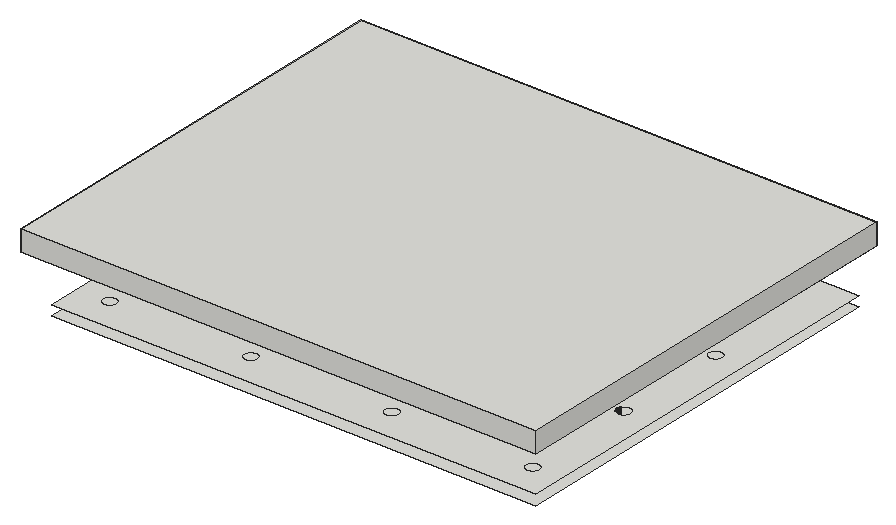
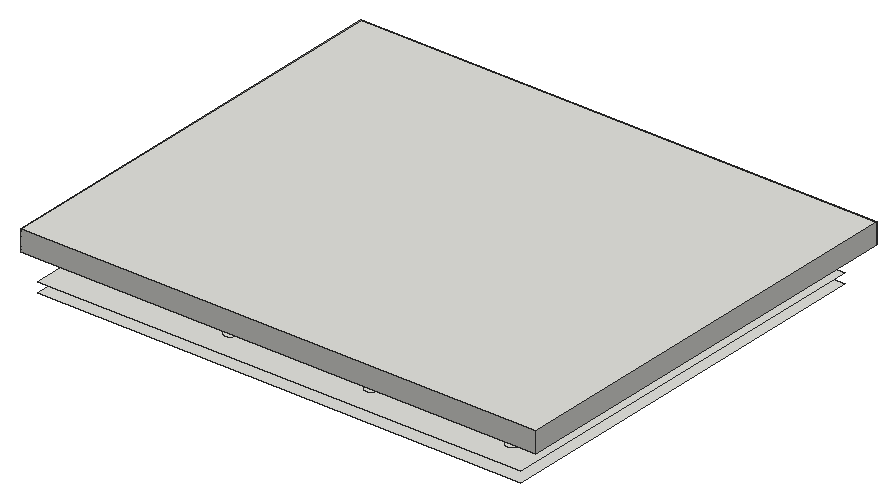
# SketchUp Ruby script. Lengths in millimetres.
U = 1.mm
M = Sketchup.active_model
def pt(a) = Geom::Point3d.new(a.map { |v| v * U })
def face(e, loops, mat)
  f = e.add_face(loops[0].map { |a| pt(a) })
  loops[1..].each { |l| e.add_face(l.map { |a| pt(a) }).erase! }
  f.material = f.back_material = mat if mat
  f
end
# faces: each face lists its corners as indices into pts; further lists are holes
def faces(e, pts, list, mat = nil) = list.each { |f| face(e, (f[0].is_a?(Array) ? f : [f]).map { |l| l.map { |i| pts[i] } }, mat) }
# xy, xz, yz: faces in a plane at the given z, y or x. An outline is a flat list of corners, or four numbers for a rectangle; further outlines are holes
def ring(l) = l.size == 4 ? [[l[0], l[1]], [l[2], l[1]], [l[2], l[3]], [l[0], l[3]]] : l.each_slice(2).to_a
def flat(e, list, mat, &to3) = list.each { |f| face(e, (f[0].is_a?(Array) ? f : [f]).map { |l| ring(l).map { |u, v| to3.(u, v) } }, mat) }
def xy(e, z, list, mat = nil) = flat(e, list, mat) { |x, y| [x, y, z] }
def xz(e, y, list, mat = nil) = flat(e, list, mat) { |x, z| [x, y, z] }
def yz(e, x, list, mat = nil) = flat(e, list, mat) { |y, z| [x, y, z] }
def lines(e, pts, list) = list.each { |a, b| e.add_line(pt(pts[a]), pt(pts[b])) }
# prism: a flat outline (further loops are holes) pulled along v
def prism(e, loops, v, mat = nil)
  f = face(e, loops, mat); d = Geom::Vector3d.new(v.map { |x| x * U })
  f.pushpull(f.normal.samedirection?(d) ? d.length : -d.length)
end
def box(e, o, s, mat = nil) = prism(e, [[o, [o[0] + s[0], o[1], o[2]], [o[0] + s[0], o[1] + s[1], o[2]], [o[0], o[1] + s[1], o[2]]]], [0, 0, s[2]], mat)
def at(x, y, z, deg = 0) = Geom::Transformation.translation(pt([x, y, z])) * Geom::Transformation.rotation(ORIGIN, Z_AXIS, deg.degrees)
def axes(o, x, y, z) = Geom::Transformation.new([*x, 0, *y, 0, *z, 0, *pt(o).to_a, 1])
def part(name) = M.definitions.add(name)
# library, detail: a bought-in or finely detailed component or shape, given as its bounding box
def library(name, o, s) = part(name).tap { |d| box(d.entities, o, s) }
def detail(e, o, s) = box(e.add_group.entities, o, s)
def put(e, d, t, mat = nil) = e.add_instance(d, t).tap { |i| i.material = mat if mat }
def group(e, t, mat = nil) = e.add_group.tap { |g| g.transformation = t; g.material = mat if mat }.entities
root = M.entities
c1 = part("Group\#21")
box(c1.entities,[-2669.7,0,0],[3683.6,3048,150])
xy(root,2718.2,[[[228.6,0,3683.6,2895.6],[685.8,457.2,3226.4,2438.4],[1465.5,177.8,1468.7,177.9,1471.9,178.2,1475.1,178.7,1478.2,179.4,1481.2,180.3,1484.2,181.4,1487.2,182.6,1490,184.1,1492.8,185.7,1495.4,187.5,1497.9,189.5,1500.3,191.6,1502.6,193.8,1504.7,196.2,1506.6,198.7,1508.4,201.4,1510,204.1,1511.5,207,1512.8,209.9,1513.8,212.9,1514.7,216,1515.4,219.1,1515.9,222.2,1516.2,225.4,1516.3,228.6,1516.2,231.8,1515.9,235,1515.4,238.1,1514.7,241.2,1513.8,244.3,1512.8,247.3,1511.5,250.2,1510,253.1,1508.4,255.8,1506.6,258.5,1504.7,261,1502.6,263.4,1500.3,265.6,1497.9,267.7,1495.4,269.7,1492.8,271.5,1490,273.1,1487.2,274.6,1484.2,275.8,1481.2,276.9,1478.2,277.8,1475.1,278.5,1471.9,279,1468.7,279.3,1465.5,279.4,1462.3,279.3,1459.2,279,1456,278.5,1452.9,277.8,1449.8,276.9,1446.8,275.8,1443.9,274.6,1441.1,273.1,1438.3,271.5,1435.7,269.7,1433.2,267.7,1430.8,265.6,1428.5,263.4,1426.4,261,1424.4,258.5,1422.6,255.8,1421,253.1,1419.6,250.2,1418.3,247.3,1417.2,244.3,1416.3,241.2,1415.6,238.1,1415.1,235,1414.8,231.8,1414.7,228.6,1414.8,225.4,1415.1,222.2,1415.6,219.1,1416.3,216,1417.2,212.9,1418.3,209.9,1419.6,207,1421,204.1,1422.6,201.4,1424.4,198.7,1426.4,196.2,1428.5,193.8,1430.8,191.6,1433.2,189.5,1435.7,187.5,1438.3,185.7,1441.1,184.1,1443.9,182.6,1446.8,181.4,1449.8,180.3,1452.9,179.4,1456,178.7,1459.2,178.2,1462.3,177.9],[457.2,177.8,460.4,177.9,463.6,178.2,466.7,178.7,469.8,179.4,472.9,180.3,475.9,181.4,478.8,182.6,481.7,184.1,484.4,185.7,487.1,187.5,489.6,189.5,492,191.6,494.2,193.8,496.3,196.2,498.3,198.7,500.1,201.4,501.7,204.1,503.2,207,504.4,209.9,505.5,212.9,506.4,216,507.1,219.1,507.6,222.2,507.9,225.4,508,228.6,507.9,231.8,507.6,235,507.1,238.1,506.4,241.2,505.5,244.3,504.4,247.3,503.2,250.2,501.7,253.1,500.1,255.8,498.3,258.5,496.3,261,494.2,263.4,492,265.6,489.6,267.7,487.1,269.7,484.4,271.5,481.7,273.1,478.8,274.6,475.9,275.8,472.9,276.9,469.8,277.8,466.7,278.5,463.6,279,460.4,279.3,457.2,279.4,454,279.3,450.8,279,447.7,278.5,444.6,277.8,441.5,276.9,438.5,275.8,435.6,274.6,432.7,273.1,430,271.5,427.3,269.7,424.8,267.7,422.4,265.6,420.2,263.4,418.1,261,416.1,258.5,414.3,255.8,412.7,253.1,411.2,250.2,410,247.3,408.9,244.3,408,241.2,407.3,238.1,406.8,235,406.5,231.8,406.4,228.6,406.5,225.4,406.8,222.2,407.3,219.1,408,216,408.9,212.9,410,209.9,411.2,207,412.7,204.1,414.3,201.4,416.1,198.7,418.1,196.2,420.2,193.8,422.4,191.6,424.8,189.5,427.3,187.5,430,185.7,432.7,184.1,435.6,182.6,438.5,181.4,441.5,180.3,444.6,179.4,447.7,178.7,450.8,178.2,454,177.9],[2473.9,177.8,2477.1,177.9,2480.2,178.2,2483.4,178.7,2486.5,179.4,2489.6,180.3,2492.6,181.4,2495.5,182.6,2498.3,184.1,2501.1,185.7,2503.7,187.5,2506.2,189.5,2508.6,191.6,2510.9,193.8,2513,196.2,2515,198.7,2516.8,201.4,2518.4,204.1,2519.8,207,2521.1,209.9,2522.2,212.9,2523.1,216,2523.8,219.1,2524.3,222.2,2524.6,225.4,2524.7,228.6,2524.6,231.8,2524.3,235,2523.8,238.1,2523.1,241.2,2522.2,244.3,2521.1,247.3,2519.8,250.2,2518.4,253.1,2516.8,255.8,2515,258.5,2513,261,2510.9,263.4,2508.6,265.6,2506.2,267.7,2503.7,269.7,2501.1,271.5,2498.3,273.1,2495.5,274.6,2492.6,275.8,2489.6,276.9,2486.5,277.8,2483.4,278.5,2480.2,279,2477.1,279.3,2473.9,279.4,2470.7,279.3,2467.5,279,2464.3,278.5,2461.2,277.8,2458.2,276.9,2455.2,275.8,2452.2,274.6,2449.4,273.1,2446.6,271.5,2444,269.7,2441.5,267.7,2439.1,265.6,2436.8,263.4,2434.7,261,2432.8,258.5,2431,255.8,2429.4,253.1,2427.9,250.2,2426.6,247.3,2425.6,244.3,2424.7,241.2,2424,238.1,2423.5,235,2423.2,231.8,2423.1,228.6,2423.2,225.4,2423.5,222.2,2424,219.1,2424.7,216,2425.6,212.9,2426.6,209.9,2427.9,207,2429.4,204.1,2431,201.4,2432.8,198.7,2434.7,196.2,2436.8,193.8,2439.1,191.6,2441.5,189.5,2444,187.5,2446.6,185.7,2449.4,184.1,2452.2,182.6,2455.2,181.4,2458.2,180.3,2461.2,179.4,2464.3,178.7,2467.5,178.2,2470.7,177.9],[3482.2,995.5,3485.4,995.6,3488.6,995.9,3491.7,996.4,3494.8,997.1,3497.9,998,3500.9,999,3503.8,1000.3,3506.7,1001.8,3509.4,1003.4,3512.1,1005.2,3514.6,1007.1,3517,1009.2,3519.2,1011.5,3521.3,1013.9,3523.3,1016.4,3525.1,1019,3526.7,1021.8,3528.2,1024.6,3529.4,1027.6,3530.5,1030.6,3531.4,1033.6,3532.1,1036.7,3532.6,1039.9,3532.9,1043.1,3533,1046.3,3532.9,1049.5,3532.6,1052.6,3532.1,1055.8,3531.4,1058.9,3530.5,1062,3529.4,1065,3528.2,1067.9,3526.7,1070.7,3525.1,1073.5,3523.3,1076.1,3521.3,1078.6,3519.2,1081,3517,1083.3,3514.6,1085.4,3512.1,1087.4,3509.4,1089.2,3506.7,1090.8,3503.8,1092.2,3500.9,1093.5,3497.9,1094.6,3494.8,1095.5,3491.7,1096.2,3488.6,1096.7,3485.4,1097,3482.2,1097.1,3479,1097,3475.8,1096.7,3472.7,1096.2,3469.6,1095.5,3466.5,1094.6,3463.5,1093.5,3460.6,1092.2,3457.7,1090.8,3455,1089.2,3452.3,1087.4,3449.8,1085.4,3447.4,1083.3,3445.2,1081,3443.1,1078.6,3441.1,1076.1,3439.3,1073.5,3437.7,1070.7,3436.2,1067.9,3435,1065,3433.9,1062,3433,1058.9,3432.3,1055.8,3431.8,1052.6,3431.5,1049.5,3431.4,1046.3,3431.5,1043.1,3431.8,1039.9,3432.3,1036.7,3433,1033.6,3433.9,1030.6,3435,1027.6,3436.2,1024.6,3437.7,1021.8,3439.3,1019,3441.1,1016.4,3443.1,1013.9,3445.2,1011.5,3447.4,1009.2,3449.8,1007.1,3452.3,1005.2,3455,1003.4,3457.7,1001.8,3460.6,1000.3,3463.5,999,3466.5,998,3469.6,997.1,3472.7,996.4,3475.8,995.9,3479,995.6],[457.2,1813.1,460.4,1813.2,463.6,1813.5,466.7,1814,469.8,1814.7,472.9,1815.6,475.9,1816.7,478.8,1818,481.7,1819.4,484.4,1821,487.1,1822.8,489.6,1824.8,492,1826.9,494.2,1829.2,496.3,1831.6,498.3,1834.1,500.1,1836.7,501.7,1839.5,503.2,1842.3,504.4,1845.2,505.5,1848.2,506.4,1851.3,507.1,1854.4,507.6,1857.6,507.9,1860.7,508,1863.9,507.9,1867.1,507.6,1870.3,507.1,1873.5,506.4,1876.6,505.5,1879.6,504.4,1882.6,503.2,1885.6,501.7,1888.4,500.1,1891.2,498.3,1893.8,496.3,1896.3,494.2,1898.7,492,1901,489.6,1903.1,487.1,1905,484.4,1906.8,481.7,1908.4,478.8,1909.9,475.9,1911.2,472.9,1912.2,469.8,1913.1,466.7,1913.8,463.6,1914.3,460.4,1914.6,457.2,1914.7,454,1914.6,450.8,1914.3,447.7,1913.8,444.6,1913.1,441.5,1912.2,438.5,1911.2,435.6,1909.9,432.7,1908.4,430,1906.8,427.3,1905,424.8,1903.1,422.4,1901,420.2,1898.7,418.1,1896.3,416.1,1893.8,414.3,1891.2,412.7,1888.4,411.2,1885.6,410,1882.6,408.9,1879.6,408,1876.6,407.3,1873.5,406.8,1870.3,406.5,1867.1,406.4,1863.9,406.5,1860.7,406.8,1857.6,407.3,1854.4,408,1851.3,408.9,1848.2,410,1845.2,411.2,1842.3,412.7,1839.5,414.3,1836.7,416.1,1834.1,418.1,1831.6,420.2,1829.2,422.4,1826.9,424.8,1824.8,427.3,1822.8,430,1821,432.7,1819.4,435.6,1818,438.5,1816.7,441.5,1815.6,444.6,1814.7,447.7,1814,450.8,1813.5,454,1813.2],[457.2,995.5,460.4,995.6,463.6,995.9,466.7,996.4,469.8,997.1,472.9,998,475.9,999,478.8,1000.3,481.7,1001.8,484.4,1003.4,487.1,1005.2,489.6,1007.1,492,1009.2,494.2,1011.5,496.3,1013.9,498.3,1016.4,500.1,1019,501.7,1021.8,503.2,1024.6,504.4,1027.6,505.5,1030.6,506.4,1033.6,507.1,1036.7,507.6,1039.9,507.9,1043.1,508,1046.3,507.9,1049.5,507.6,1052.6,507.1,1055.8,506.4,1058.9,505.5,1062,504.4,1065,503.2,1067.9,501.7,1070.7,500.1,1073.5,498.3,1076.1,496.3,1078.6,494.2,1081,492,1083.3,489.6,1085.4,487.1,1087.4,484.4,1089.2,481.7,1090.8,478.8,1092.2,475.9,1093.5,472.9,1094.6,469.8,1095.5,466.7,1096.2,463.6,1096.7,460.4,1097,457.2,1097.1,454,1097,450.8,1096.7,447.7,1096.2,444.6,1095.5,441.5,1094.6,438.5,1093.5,435.6,1092.2,432.7,1090.8,430,1089.2,427.3,1087.4,424.8,1085.4,422.4,1083.3,420.2,1081,418.1,1078.6,416.1,1076.1,414.3,1073.5,412.7,1070.7,411.2,1067.9,410,1065,408.9,1062,408,1058.9,407.3,1055.8,406.8,1052.6,406.5,1049.5,406.4,1046.3,406.5,1043.1,406.8,1039.9,407.3,1036.7,408,1033.6,408.9,1030.6,410,1027.6,411.2,1024.6,412.7,1021.8,414.3,1019,416.1,1016.4,418.1,1013.9,420.2,1011.5,422.4,1009.2,424.8,1007.1,427.3,1005.2,430,1003.4,432.7,1001.8,435.6,1000.3,438.5,999,441.5,998,444.6,997.1,447.7,996.4,450.8,995.9,454,995.6],[3482.2,177.8,3485.4,177.9,3488.6,178.2,3491.7,178.7,3494.8,179.4,3497.9,180.3,3500.9,181.4,3503.8,182.6,3506.7,184.1,3509.4,185.7,3512.1,187.5,3514.6,189.5,3517,191.6,3519.2,193.8,3521.3,196.2,3523.3,198.7,3525.1,201.4,3526.7,204.1,3528.2,207,3529.4,209.9,3530.5,212.9,3531.4,216,3532.1,219.1,3532.6,222.2,3532.9,225.4,3533,228.6,3532.9,231.8,3532.6,235,3532.1,238.1,3531.4,241.2,3530.5,244.3,3529.4,247.3,3528.2,250.2,3526.7,253.1,3525.1,255.8,3523.3,258.5,3521.3,261,3519.2,263.4,3517,265.6,3514.6,267.7,3512.1,269.7,3509.4,271.5,3506.7,273.1,3503.8,274.6,3500.9,275.8,3497.9,276.9,3494.8,277.8,3491.7,278.5,3488.6,279,3485.4,279.3,3482.2,279.4,3479,279.3,3475.8,279,3472.7,278.5,3469.6,277.8,3466.5,276.9,3463.5,275.8,3460.6,274.6,3457.7,273.1,3455,271.5,3452.3,269.7,3449.8,267.7,3447.4,265.6,3445.2,263.4,3443.1,261,3441.1,258.5,3439.3,255.8,3437.7,253.1,3436.2,250.2,3435,247.3,3433.9,244.3,3433,241.2,3432.3,238.1,3431.8,235,3431.5,231.8,3431.4,228.6,3431.5,225.4,3431.8,222.2,3432.3,219.1,3433,216,3433.9,212.9,3435,209.9,3436.2,207,3437.7,204.1,3439.3,201.4,3441.1,198.7,3443.1,196.2,3445.2,193.8,3447.4,191.6,3449.8,189.5,3452.3,187.5,3455,185.7,3457.7,184.1,3460.6,182.6,3463.5,181.4,3466.5,180.3,3469.6,179.4,3472.7,178.7,3475.8,178.2,3479,177.9],[457.2,2630.8,460.4,2630.9,463.6,2631.2,466.7,2631.7,469.8,2632.4,472.9,2633.3,475.9,2634.4,478.8,2635.6,481.7,2637.1,484.4,2638.7,487.1,2640.5,489.6,2642.5,492,2644.6,494.2,2646.8,496.3,2649.2,498.3,2651.7,500.1,2654.4,501.7,2657.1,503.2,2660,504.4,2662.9,505.5,2665.9,506.4,2669,507.1,2672.1,507.6,2675.2,507.9,2678.4,508,2681.6,507.9,2684.8,507.6,2688,507.1,2691.1,506.4,2694.2,505.5,2697.3,504.4,2700.3,503.2,2703.2,501.7,2706.1,500.1,2708.8,498.3,2711.5,496.3,2714,494.2,2716.4,492,2718.6,489.6,2720.7,487.1,2722.7,484.4,2724.5,481.7,2726.1,478.8,2727.6,475.9,2728.8,472.9,2729.9,469.8,2730.8,466.7,2731.5,463.6,2732,460.4,2732.3,457.2,2732.4,454,2732.3,450.8,2732,447.7,2731.5,444.6,2730.8,441.5,2729.9,438.5,2728.8,435.6,2727.6,432.7,2726.1,430,2724.5,427.3,2722.7,424.8,2720.7,422.4,2718.6,420.2,2716.4,418.1,2714,416.1,2711.5,414.3,2708.8,412.7,2706.1,411.2,2703.2,410,2700.3,408.9,2697.3,408,2694.2,407.3,2691.1,406.8,2688,406.5,2684.8,406.4,2681.6,406.5,2678.4,406.8,2675.2,407.3,2672.1,408,2669,408.9,2665.9,410,2662.9,411.2,2660,412.7,2657.1,414.3,2654.4,416.1,2651.7,418.1,2649.2,420.2,2646.8,422.4,2644.6,424.8,2642.5,427.3,2640.5,430,2638.7,432.7,2637.1,435.6,2635.6,438.5,2634.4,441.5,2633.3,444.6,2632.4,447.7,2631.7,450.8,2631.2,454,2630.9],[2473.9,2630.8,2477.1,2630.9,2480.2,2631.2,2483.4,2631.7,2486.5,2632.4,2489.6,2633.3,2492.6,2634.4,2495.5,2635.6,2498.3,2637.1,2501.1,2638.7,2503.7,2640.5,2506.2,2642.5,2508.6,2644.6,2510.9,2646.8,2513,2649.2,2515,2651.7,2516.8,2654.4,2518.4,2657.1,2519.8,2660,2521.1,2662.9,2522.2,2665.9,2523.1,2669,2523.8,2672.1,2524.3,2675.2,2524.6,2678.4,2524.7,2681.6,2524.6,2684.8,2524.3,2688,2523.8,2691.1,2523.1,2694.2,2522.2,2697.3,2521.1,2700.3,2519.8,2703.2,2518.4,2706.1,2516.8,2708.8,2515,2711.5,2513,2714,2510.9,2716.4,2508.6,2718.6,2506.2,2720.7,2503.7,2722.7,2501.1,2724.5,2498.3,2726.1,2495.5,2727.6,2492.6,2728.8,2489.6,2729.9,2486.5,2730.8,2483.4,2731.5,2480.2,2732,2477.1,2732.3,2473.9,2732.4,2470.7,2732.3,2467.5,2732,2464.3,2731.5,2461.2,2730.8,2458.2,2729.9,2455.2,2728.8,2452.2,2727.6,2449.4,2726.1,2446.6,2724.5,2444,2722.7,2441.5,2720.7,2439.1,2718.6,2436.8,2716.4,2434.7,2714,2432.8,2711.5,2431,2708.8,2429.4,2706.1,2427.9,2703.2,2426.6,2700.3,2425.6,2697.3,2424.7,2694.2,2424,2691.1,2423.5,2688,2423.2,2684.8,2423.1,2681.6,2423.2,2678.4,2423.5,2675.2,2424,2672.1,2424.7,2669,2425.6,2665.9,2426.6,2662.9,2427.9,2660,2429.4,2657.1,2431,2654.4,2432.8,2651.7,2434.7,2649.2,2436.8,2646.8,2439.1,2644.6,2441.5,2642.5,2444,2640.5,2446.6,2638.7,2449.4,2637.1,2452.2,2635.6,2455.2,2634.4,2458.2,2633.3,2461.2,2632.4,2464.3,2631.7,2467.5,2631.2,2470.7,2630.9],[1465.5,2630.8,1468.7,2630.9,1471.9,2631.2,1475.1,2631.7,1478.2,2632.4,1481.2,2633.3,1484.2,2634.4,1487.2,2635.6,1490,2637.1,1492.8,2638.7,1495.4,2640.5,1497.9,2642.5,1500.3,2644.6,1502.6,2646.8,1504.7,2649.2,1506.6,2651.7,1508.4,2654.4,1510,2657.1,1511.5,2660,1512.8,2662.9,1513.8,2665.9,1514.7,2669,1515.4,2672.1,1515.9,2675.2,1516.2,2678.4,1516.3,2681.6,1516.2,2684.8,1515.9,2688,1515.4,2691.1,1514.7,2694.2,1513.8,2697.3,1512.8,2700.3,1511.5,2703.2,1510,2706.1,1508.4,2708.8,1506.6,2711.5,1504.7,2714,1502.6,2716.4,1500.3,2718.6,1497.9,2720.7,1495.4,2722.7,1492.8,2724.5,1490,2726.1,1487.2,2727.6,1484.2,2728.8,1481.2,2729.9,1478.2,2730.8,1475.1,2731.5,1471.9,2732,1468.7,2732.3,1465.5,2732.4,1462.3,2732.3,1459.2,2732,1456,2731.5,1452.9,2730.8,1449.8,2729.9,1446.8,2728.8,1443.9,2727.6,1441.1,2726.1,1438.3,2724.5,1435.7,2722.7,1433.2,2720.7,1430.8,2718.6,1428.5,2716.4,1426.4,2714,1424.4,2711.5,1422.6,2708.8,1421,2706.1,1419.6,2703.2,1418.3,2700.3,1417.2,2697.3,1416.3,2694.2,1415.6,2691.1,1415.1,2688,1414.8,2684.8,1414.7,2681.6,1414.8,2678.4,1415.1,2675.2,1415.6,2672.1,1416.3,2669,1417.2,2665.9,1418.3,2662.9,1419.6,2660,1421,2657.1,1422.6,2654.4,1424.4,2651.7,1426.4,2649.2,1428.5,2646.8,1430.8,2644.6,1433.2,2642.5,1435.7,2640.5,1438.3,2638.7,1441.1,2637.1,1443.9,2635.6,1446.8,2634.4,1449.8,2633.3,1452.9,2632.4,1456,2631.7,1459.2,2631.2,1462.3,2630.9],[3482.2,1813.1,3485.4,1813.2,3488.6,1813.5,3491.7,1814,3494.8,1814.7,3497.9,1815.6,3500.9,1816.7,3503.8,1818,3506.7,1819.4,3509.4,1821,3512.1,1822.8,3514.6,1824.8,3517,1826.9,3519.2,1829.2,3521.3,1831.6,3523.3,1834.1,3525.1,1836.7,3526.7,1839.5,3528.2,1842.3,3529.4,1845.2,3530.5,1848.2,3531.4,1851.3,3532.1,1854.4,3532.6,1857.6,3532.9,1860.7,3533,1863.9,3532.9,1867.1,3532.6,1870.3,3532.1,1873.5,3531.4,1876.6,3530.5,1879.6,3529.4,1882.6,3528.2,1885.6,3526.7,1888.4,3525.1,1891.2,3523.3,1893.8,3521.3,1896.3,3519.2,1898.7,3517,1901,3514.6,1903.1,3512.1,1905,3509.4,1906.8,3506.7,1908.4,3503.8,1909.9,3500.9,1911.2,3497.9,1912.2,3494.8,1913.1,3491.7,1913.8,3488.6,1914.3,3485.4,1914.6,3482.2,1914.7,3479,1914.6,3475.8,1914.3,3472.7,1913.8,3469.6,1913.1,3466.5,1912.2,3463.5,1911.2,3460.6,1909.9,3457.7,1908.4,3455,1906.8,3452.3,1905,3449.8,1903.1,3447.4,1901,3445.2,1898.7,3443.1,1896.3,3441.1,1893.8,3439.3,1891.2,3437.7,1888.4,3436.2,1885.6,3435,1882.6,3433.9,1879.6,3433,1876.6,3432.3,1873.5,3431.8,1870.3,3431.5,1867.1,3431.4,1863.9,3431.5,1860.7,3431.8,1857.6,3432.3,1854.4,3433,1851.3,3433.9,1848.2,3435,1845.2,3436.2,1842.3,3437.7,1839.5,3439.3,1836.7,3441.1,1834.1,3443.1,1831.6,3445.2,1829.2,3447.4,1826.9,3449.8,1824.8,3452.3,1822.8,3455,1821,3457.7,1819.4,3460.6,1818,3463.5,1816.7,3466.5,1815.6,3469.6,1814.7,3472.7,1814,3475.8,1813.5,3479,1813.2]]])
xy(root,2743.2,[[[635,406.4,3277.2,2489.2],[673.1,444.5,3239.1,2451.1]],[[1003.3,774.7,2908.9,2120.9],[1041.4,812.8,2870.8,2082.8]]])
xy(root,2766.6,[[[673.1,444.5,3239.1,2451.1],[685.8,457.2,3226.4,2438.4]]])
xy(root,2768.6,[[[990.6,762,2921.6,2133.6],[1003.3,774.7,2908.9,2120.9]]])
xy(root,2794,[[[228.6,0,3683.6,2895.6],[635,406.4,3277.2,2489.2],[457.2,1813.1,454,1813.2,450.8,1813.5,447.7,1814,444.6,1814.7,441.5,1815.6,438.5,1816.7,435.6,1818,432.7,1819.4,430,1821,427.3,1822.8,424.8,1824.8,422.4,1826.9,420.2,1829.2,418.1,1831.6,416.1,1834.1,414.3,1836.7,412.7,1839.5,411.2,1842.3,410,1845.2,408.9,1848.2,408,1851.3,407.3,1854.4,406.8,1857.6,406.5,1860.7,406.4,1863.9,406.5,1867.1,406.8,1870.3,407.3,1873.5,408,1876.6,408.9,1879.6,410,1882.6,411.2,1885.6,412.7,1888.4,414.3,1891.2,416.1,1893.8,418.1,1896.3,420.2,1898.7,422.4,1901,424.8,1903.1,427.3,1905,430,1906.8,432.7,1908.4,435.6,1909.9,438.5,1911.2,441.5,1912.2,444.6,1913.1,447.7,1913.8,450.8,1914.3,454,1914.6,457.2,1914.7,460.4,1914.6,463.6,1914.3,466.7,1913.8,469.8,1913.1,472.9,1912.2,475.9,1911.2,478.8,1909.9,481.7,1908.4,484.4,1906.8,487.1,1905,489.6,1903.1,492,1901,494.2,1898.7,496.3,1896.3,498.3,1893.8,500.1,1891.2,501.7,1888.4,503.2,1885.6,504.4,1882.6,505.5,1879.6,506.4,1876.6,507.1,1873.5,507.6,1870.3,507.9,1867.1,508,1863.9,507.9,1860.7,507.6,1857.6,507.1,1854.4,506.4,1851.3,505.5,1848.2,504.4,1845.2,503.2,1842.3,501.7,1839.5,500.1,1836.7,498.3,1834.1,496.3,1831.6,494.2,1829.2,492,1826.9,489.6,1824.8,487.1,1822.8,484.4,1821,481.7,1819.4,478.8,1818,475.9,1816.7,472.9,1815.6,469.8,1814.7,466.7,1814,463.6,1813.5,460.4,1813.2],[3482.2,177.8,3479,177.9,3475.8,178.2,3472.7,178.7,3469.6,179.4,3466.5,180.3,3463.5,181.4,3460.6,182.6,3457.7,184.1,3455,185.7,3452.3,187.5,3449.8,189.5,3447.4,191.6,3445.2,193.8,3443.1,196.2,3441.1,198.7,3439.3,201.4,3437.7,204.1,3436.2,207,3435,209.9,3433.9,212.9,3433,216,3432.3,219.1,3431.8,222.2,3431.5,225.4,3431.4,228.6,3431.5,231.8,3431.8,235,3432.3,238.1,3433,241.2,3433.9,244.3,3435,247.3,3436.2,250.2,3437.7,253.1,3439.3,255.8,3441.1,258.5,3443.1,261,3445.2,263.4,3447.4,265.6,3449.8,267.7,3452.3,269.7,3455,271.5,3457.7,273.1,3460.6,274.6,3463.5,275.8,3466.5,276.9,3469.6,277.8,3472.7,278.5,3475.8,279,3479,279.3,3482.2,279.4,3485.4,279.3,3488.6,279,3491.7,278.5,3494.8,277.8,3497.9,276.9,3500.9,275.8,3503.8,274.6,3506.7,273.1,3509.4,271.5,3512.1,269.7,3514.6,267.7,3517,265.6,3519.2,263.4,3521.3,261,3523.3,258.5,3525.1,255.8,3526.7,253.1,3528.2,250.2,3529.4,247.3,3530.5,244.3,3531.4,241.2,3532.1,238.1,3532.6,235,3532.9,231.8,3533,228.6,3532.9,225.4,3532.6,222.2,3532.1,219.1,3531.4,216,3530.5,212.9,3529.4,209.9,3528.2,207,3526.7,204.1,3525.1,201.4,3523.3,198.7,3521.3,196.2,3519.2,193.8,3517,191.6,3514.6,189.5,3512.1,187.5,3509.4,185.7,3506.7,184.1,3503.8,182.6,3500.9,181.4,3497.9,180.3,3494.8,179.4,3491.7,178.7,3488.6,178.2,3485.4,177.9],[457.2,177.8,454,177.9,450.8,178.2,447.7,178.7,444.6,179.4,441.5,180.3,438.5,181.4,435.6,182.6,432.7,184.1,430,185.7,427.3,187.5,424.8,189.5,422.4,191.6,420.2,193.8,418.1,196.2,416.1,198.7,414.3,201.4,412.7,204.1,411.2,207,410,209.9,408.9,212.9,408,216,407.3,219.1,406.8,222.2,406.5,225.4,406.4,228.6,406.5,231.8,406.8,235,407.3,238.1,408,241.2,408.9,244.3,410,247.3,411.2,250.2,412.7,253.1,414.3,255.8,416.1,258.5,418.1,261,420.2,263.4,422.4,265.6,424.8,267.7,427.3,269.7,430,271.5,432.7,273.1,435.6,274.6,438.5,275.8,441.5,276.9,444.6,277.8,447.7,278.5,450.8,279,454,279.3,457.2,279.4,460.4,279.3,463.6,279,466.7,278.5,469.8,277.8,472.9,276.9,475.9,275.8,478.8,274.6,481.7,273.1,484.4,271.5,487.1,269.7,489.6,267.7,492,265.6,494.2,263.4,496.3,261,498.3,258.5,500.1,255.8,501.7,253.1,503.2,250.2,504.4,247.3,505.5,244.3,506.4,241.2,507.1,238.1,507.6,235,507.9,231.8,508,228.6,507.9,225.4,507.6,222.2,507.1,219.1,506.4,216,505.5,212.9,504.4,209.9,503.2,207,501.7,204.1,500.1,201.4,498.3,198.7,496.3,196.2,494.2,193.8,492,191.6,489.6,189.5,487.1,187.5,484.4,185.7,481.7,184.1,478.8,182.6,475.9,181.4,472.9,180.3,469.8,179.4,466.7,178.7,463.6,178.2,460.4,177.9],[1465.5,177.8,1462.3,177.9,1459.2,178.2,1456,178.7,1452.9,179.4,1449.8,180.3,1446.8,181.4,1443.9,182.6,1441.1,184.1,1438.3,185.7,1435.7,187.5,1433.2,189.5,1430.8,191.6,1428.5,193.8,1426.4,196.2,1424.4,198.7,1422.6,201.4,1421,204.1,1419.6,207,1418.3,209.9,1417.2,212.9,1416.3,216,1415.6,219.1,1415.1,222.2,1414.8,225.4,1414.7,228.6,1414.8,231.8,1415.1,235,1415.6,238.1,1416.3,241.2,1417.2,244.3,1418.3,247.3,1419.6,250.2,1421,253.1,1422.6,255.8,1424.4,258.5,1426.4,261,1428.5,263.4,1430.8,265.6,1433.2,267.7,1435.7,269.7,1438.3,271.5,1441.1,273.1,1443.9,274.6,1446.8,275.8,1449.8,276.9,1452.9,277.8,1456,278.5,1459.2,279,1462.3,279.3,1465.5,279.4,1468.7,279.3,1471.9,279,1475.1,278.5,1478.2,277.8,1481.2,276.9,1484.2,275.8,1487.2,274.6,1490,273.1,1492.8,271.5,1495.4,269.7,1497.9,267.7,1500.3,265.6,1502.6,263.4,1504.7,261,1506.6,258.5,1508.4,255.8,1510,253.1,1511.5,250.2,1512.8,247.3,1513.8,244.3,1514.7,241.2,1515.4,238.1,1515.9,235,1516.2,231.8,1516.3,228.6,1516.2,225.4,1515.9,222.2,1515.4,219.1,1514.7,216,1513.8,212.9,1512.8,209.9,1511.5,207,1510,204.1,1508.4,201.4,1506.6,198.7,1504.7,196.2,1502.6,193.8,1500.3,191.6,1497.9,189.5,1495.4,187.5,1492.8,185.7,1490,184.1,1487.2,182.6,1484.2,181.4,1481.2,180.3,1478.2,179.4,1475.1,178.7,1471.9,178.2,1468.7,177.9],[2473.9,177.8,2470.7,177.9,2467.5,178.2,2464.3,178.7,2461.2,179.4,2458.2,180.3,2455.2,181.4,2452.2,182.6,2449.4,184.1,2446.6,185.7,2444,187.5,2441.5,189.5,2439.1,191.6,2436.8,193.8,2434.7,196.2,2432.8,198.7,2431,201.4,2429.4,204.1,2427.9,207,2426.6,209.9,2425.6,212.9,2424.7,216,2424,219.1,2423.5,222.2,2423.2,225.4,2423.1,228.6,2423.2,231.8,2423.5,235,2424,238.1,2424.7,241.2,2425.6,244.3,2426.6,247.3,2427.9,250.2,2429.4,253.1,2431,255.8,2432.8,258.5,2434.7,261,2436.8,263.4,2439.1,265.6,2441.5,267.7,2444,269.7,2446.6,271.5,2449.4,273.1,2452.2,274.6,2455.2,275.8,2458.2,276.9,2461.2,277.8,2464.3,278.5,2467.5,279,2470.7,279.3,2473.9,279.4,2477.1,279.3,2480.2,279,2483.4,278.5,2486.5,277.8,2489.6,276.9,2492.6,275.8,2495.5,274.6,2498.3,273.1,2501.1,271.5,2503.7,269.7,2506.2,267.7,2508.6,265.6,2510.9,263.4,2513,261,2515,258.5,2516.8,255.8,2518.4,253.1,2519.8,250.2,2521.1,247.3,2522.2,244.3,2523.1,241.2,2523.8,238.1,2524.3,235,2524.6,231.8,2524.7,228.6,2524.6,225.4,2524.3,222.2,2523.8,219.1,2523.1,216,2522.2,212.9,2521.1,209.9,2519.8,207,2518.4,204.1,2516.8,201.4,2515,198.7,2513,196.2,2510.9,193.8,2508.6,191.6,2506.2,189.5,2503.7,187.5,2501.1,185.7,2498.3,184.1,2495.5,182.6,2492.6,181.4,2489.6,180.3,2486.5,179.4,2483.4,178.7,2480.2,178.2,2477.1,177.9],[2473.9,2630.8,2470.7,2630.9,2467.5,2631.2,2464.3,2631.7,2461.2,2632.4,2458.2,2633.3,2455.2,2634.4,2452.2,2635.6,2449.4,2637.1,2446.6,2638.7,2444,2640.5,2441.5,2642.5,2439.1,2644.6,2436.8,2646.8,2434.7,2649.2,2432.8,2651.7,2431,2654.4,2429.4,2657.1,2427.9,2660,2426.6,2662.9,2425.6,2665.9,2424.7,2669,2424,2672.1,2423.5,2675.2,2423.2,2678.4,2423.1,2681.6,2423.2,2684.8,2423.5,2688,2424,2691.1,2424.7,2694.2,2425.6,2697.3,2426.6,2700.3,2427.9,2703.2,2429.4,2706.1,2431,2708.8,2432.8,2711.5,2434.7,2714,2436.8,2716.4,2439.1,2718.6,2441.5,2720.7,2444,2722.7,2446.6,2724.5,2449.4,2726.1,2452.2,2727.6,2455.2,2728.8,2458.2,2729.9,2461.2,2730.8,2464.3,2731.5,2467.5,2732,2470.7,2732.3,2473.9,2732.4,2477.1,2732.3,2480.2,2732,2483.4,2731.5,2486.5,2730.8,2489.6,2729.9,2492.6,2728.8,2495.5,2727.6,2498.3,2726.1,2501.1,2724.5,2503.7,2722.7,2506.2,2720.7,2508.6,2718.6,2510.9,2716.4,2513,2714,2515,2711.5,2516.8,2708.8,2518.4,2706.1,2519.8,2703.2,2521.1,2700.3,2522.2,2697.3,2523.1,2694.2,2523.8,2691.1,2524.3,2688,2524.6,2684.8,2524.7,2681.6,2524.6,2678.4,2524.3,2675.2,2523.8,2672.1,2523.1,2669,2522.2,2665.9,2521.1,2662.9,2519.8,2660,2518.4,2657.1,2516.8,2654.4,2515,2651.7,2513,2649.2,2510.9,2646.8,2508.6,2644.6,2506.2,2642.5,2503.7,2640.5,2501.1,2638.7,2498.3,2637.1,2495.5,2635.6,2492.6,2634.4,2489.6,2633.3,2486.5,2632.4,2483.4,2631.7,2480.2,2631.2,2477.1,2630.9],[1465.5,2630.8,1462.3,2630.9,1459.2,2631.2,1456,2631.7,1452.9,2632.4,1449.8,2633.3,1446.8,2634.4,1443.9,2635.6,1441.1,2637.1,1438.3,2638.7,1435.7,2640.5,1433.2,2642.5,1430.8,2644.6,1428.5,2646.8,1426.4,2649.2,1424.4,2651.7,1422.6,2654.4,1421,2657.1,1419.6,2660,1418.3,2662.9,1417.2,2665.9,1416.3,2669,1415.6,2672.1,1415.1,2675.2,1414.8,2678.4,1414.7,2681.6,1414.8,2684.8,1415.1,2688,1415.6,2691.1,1416.3,2694.2,1417.2,2697.3,1418.3,2700.3,1419.6,2703.2,1421,2706.1,1422.6,2708.8,1424.4,2711.5,1426.4,2714,1428.5,2716.4,1430.8,2718.6,1433.2,2720.7,1435.7,2722.7,1438.3,2724.5,1441.1,2726.1,1443.9,2727.6,1446.8,2728.8,1449.8,2729.9,1452.9,2730.8,1456,2731.5,1459.2,2732,1462.3,2732.3,1465.5,2732.4,1468.7,2732.3,1471.9,2732,1475.1,2731.5,1478.2,2730.8,1481.2,2729.9,1484.2,2728.8,1487.2,2727.6,1490,2726.1,1492.8,2724.5,1495.4,2722.7,1497.9,2720.7,1500.3,2718.6,1502.6,2716.4,1504.7,2714,1506.6,2711.5,1508.4,2708.8,1510,2706.1,1511.5,2703.2,1512.8,2700.3,1513.8,2697.3,1514.7,2694.2,1515.4,2691.1,1515.9,2688,1516.2,2684.8,1516.3,2681.6,1516.2,2678.4,1515.9,2675.2,1515.4,2672.1,1514.7,2669,1513.8,2665.9,1512.8,2662.9,1511.5,2660,1510,2657.1,1508.4,2654.4,1506.6,2651.7,1504.7,2649.2,1502.6,2646.8,1500.3,2644.6,1497.9,2642.5,1495.4,2640.5,1492.8,2638.7,1490,2637.1,1487.2,2635.6,1484.2,2634.4,1481.2,2633.3,1478.2,2632.4,1475.1,2631.7,1471.9,2631.2,1468.7,2630.9],[3482.2,995.5,3479,995.6,3475.8,995.9,3472.7,996.4,3469.6,997.1,3466.5,998,3463.5,999,3460.6,1000.3,3457.7,1001.8,3455,1003.4,3452.3,1005.2,3449.8,1007.1,3447.4,1009.2,3445.2,1011.5,3443.1,1013.9,3441.1,1016.4,3439.3,1019,3437.7,1021.8,3436.2,1024.6,3435,1027.6,3433.9,1030.6,3433,1033.6,3432.3,1036.7,3431.8,1039.9,3431.5,1043.1,3431.4,1046.3,3431.5,1049.5,3431.8,1052.6,3432.3,1055.8,3433,1058.9,3433.9,1062,3435,1065,3436.2,1067.9,3437.7,1070.7,3439.3,1073.5,3441.1,1076.1,3443.1,1078.6,3445.2,1081,3447.4,1083.3,3449.8,1085.4,3452.3,1087.4,3455,1089.2,3457.7,1090.8,3460.6,1092.2,3463.5,1093.5,3466.5,1094.6,3469.6,1095.5,3472.7,1096.2,3475.8,1096.7,3479,1097,3482.2,1097.1,3485.4,1097,3488.6,1096.7,3491.7,1096.2,3494.8,1095.5,3497.9,1094.6,3500.9,1093.5,3503.8,1092.2,3506.7,1090.8,3509.4,1089.2,3512.1,1087.4,3514.6,1085.4,3517,1083.3,3519.2,1081,3521.3,1078.6,3523.3,1076.1,3525.1,1073.5,3526.7,1070.7,3528.2,1067.9,3529.4,1065,3530.5,1062,3531.4,1058.9,3532.1,1055.8,3532.6,1052.6,3532.9,1049.5,3533,1046.3,3532.9,1043.1,3532.6,1039.9,3532.1,1036.7,3531.4,1033.6,3530.5,1030.6,3529.4,1027.6,3528.2,1024.6,3526.7,1021.8,3525.1,1019,3523.3,1016.4,3521.3,1013.9,3519.2,1011.5,3517,1009.2,3514.6,1007.1,3512.1,1005.2,3509.4,1003.4,3506.7,1001.8,3503.8,1000.3,3500.9,999,3497.9,998,3494.8,997.1,3491.7,996.4,3488.6,995.9,3485.4,995.6],[457.2,995.5,454,995.6,450.8,995.9,447.7,996.4,444.6,997.1,441.5,998,438.5,999,435.6,1000.3,432.7,1001.8,430,1003.4,427.3,1005.2,424.8,1007.1,422.4,1009.2,420.2,1011.5,418.1,1013.9,416.1,1016.4,414.3,1019,412.7,1021.8,411.2,1024.6,410,1027.6,408.9,1030.6,408,1033.6,407.3,1036.7,406.8,1039.9,406.5,1043.1,406.4,1046.3,406.5,1049.5,406.8,1052.6,407.3,1055.8,408,1058.9,408.9,1062,410,1065,411.2,1067.9,412.7,1070.7,414.3,1073.5,416.1,1076.1,418.1,1078.6,420.2,1081,422.4,1083.3,424.8,1085.4,427.3,1087.4,430,1089.2,432.7,1090.8,435.6,1092.2,438.5,1093.5,441.5,1094.6,444.6,1095.5,447.7,1096.2,450.8,1096.7,454,1097,457.2,1097.1,460.4,1097,463.6,1096.7,466.7,1096.2,469.8,1095.5,472.9,1094.6,475.9,1093.5,478.8,1092.2,481.7,1090.8,484.4,1089.2,487.1,1087.4,489.6,1085.4,492,1083.3,494.2,1081,496.3,1078.6,498.3,1076.1,500.1,1073.5,501.7,1070.7,503.2,1067.9,504.4,1065,505.5,1062,506.4,1058.9,507.1,1055.8,507.6,1052.6,507.9,1049.5,508,1046.3,507.9,1043.1,507.6,1039.9,507.1,1036.7,506.4,1033.6,505.5,1030.6,504.4,1027.6,503.2,1024.6,501.7,1021.8,500.1,1019,498.3,1016.4,496.3,1013.9,494.2,1011.5,492,1009.2,489.6,1007.1,487.1,1005.2,484.4,1003.4,481.7,1001.8,478.8,1000.3,475.9,999,472.9,998,469.8,997.1,466.7,996.4,463.6,995.9,460.4,995.6],[457.2,2630.8,454,2630.9,450.8,2631.2,447.7,2631.7,444.6,2632.4,441.5,2633.3,438.5,2634.4,435.6,2635.6,432.7,2637.1,430,2638.7,427.3,2640.5,424.8,2642.5,422.4,2644.6,420.2,2646.8,418.1,2649.2,416.1,2651.7,414.3,2654.4,412.7,2657.1,411.2,2660,410,2662.9,408.9,2665.9,408,2669,407.3,2672.1,406.8,2675.2,406.5,2678.4,406.4,2681.6,406.5,2684.8,406.8,2688,407.3,2691.1,408,2694.2,408.9,2697.3,410,2700.3,411.2,2703.2,412.7,2706.1,414.3,2708.8,416.1,2711.5,418.1,2714,420.2,2716.4,422.4,2718.6,424.8,2720.7,427.3,2722.7,430,2724.5,432.7,2726.1,435.6,2727.6,438.5,2728.8,441.5,2729.9,444.6,2730.8,447.7,2731.5,450.8,2732,454,2732.3,457.2,2732.4,460.4,2732.3,463.6,2732,466.7,2731.5,469.8,2730.8,472.9,2729.9,475.9,2728.8,478.8,2727.6,481.7,2726.1,484.4,2724.5,487.1,2722.7,489.6,2720.7,492,2718.6,494.2,2716.4,496.3,2714,498.3,2711.5,500.1,2708.8,501.7,2706.1,503.2,2703.2,504.4,2700.3,505.5,2697.3,506.4,2694.2,507.1,2691.1,507.6,2688,507.9,2684.8,508,2681.6,507.9,2678.4,507.6,2675.2,507.1,2672.1,506.4,2669,505.5,2665.9,504.4,2662.9,503.2,2660,501.7,2657.1,500.1,2654.4,498.3,2651.7,496.3,2649.2,494.2,2646.8,492,2644.6,489.6,2642.5,487.1,2640.5,484.4,2638.7,481.7,2637.1,478.8,2635.6,475.9,2634.4,472.9,2633.3,469.8,2632.4,466.7,2631.7,463.6,2631.2,460.4,2630.9],[3482.2,1813.1,3479,1813.2,3475.8,1813.5,3472.7,1814,3469.6,1814.7,3466.5,1815.6,3463.5,1816.7,3460.6,1818,3457.7,1819.4,3455,1821,3452.3,1822.8,3449.8,1824.8,3447.4,1826.9,3445.2,1829.2,3443.1,1831.6,3441.1,1834.1,3439.3,1836.7,3437.7,1839.5,3436.2,1842.3,3435,1845.2,3433.9,1848.2,3433,1851.3,3432.3,1854.4,3431.8,1857.6,3431.5,1860.7,3431.4,1863.9,3431.5,1867.1,3431.8,1870.3,3432.3,1873.5,3433,1876.6,3433.9,1879.6,3435,1882.6,3436.2,1885.6,3437.7,1888.4,3439.3,1891.2,3441.1,1893.8,3443.1,1896.3,3445.2,1898.7,3447.4,1901,3449.8,1903.1,3452.3,1905,3455,1906.8,3457.7,1908.4,3460.6,1909.9,3463.5,1911.2,3466.5,1912.2,3469.6,1913.1,3472.7,1913.8,3475.8,1914.3,3479,1914.6,3482.2,1914.7,3485.4,1914.6,3488.6,1914.3,3491.7,1913.8,3494.8,1913.1,3497.9,1912.2,3500.9,1911.2,3503.8,1909.9,3506.7,1908.4,3509.4,1906.8,3512.1,1905,3514.6,1903.1,3517,1901,3519.2,1898.7,3521.3,1896.3,3523.3,1893.8,3525.1,1891.2,3526.7,1888.4,3528.2,1885.6,3529.4,1882.6,3530.5,1879.6,3531.4,1876.6,3532.1,1873.5,3532.6,1870.3,3532.9,1867.1,3533,1863.9,3532.9,1860.7,3532.6,1857.6,3532.1,1854.4,3531.4,1851.3,3530.5,1848.2,3529.4,1845.2,3528.2,1842.3,3526.7,1839.5,3525.1,1836.7,3523.3,1834.1,3521.3,1831.6,3519.2,1829.2,3517,1826.9,3514.6,1824.8,3512.1,1822.8,3509.4,1821,3506.7,1819.4,3503.8,1818,3500.9,1816.7,3497.9,1815.6,3494.8,1814.7,3491.7,1814,3488.6,1813.5,3485.4,1813.2]],[[635,406.4,3277.2,2489.2],[1041.4,812.8,2870.8,2082.8]],[1041.4,812.8,2870.8,2082.8]])
xz(root,406.4,[[635,2743.2,3277.2,2794]])
xz(root,444.5,[[673.1,2743.2,3239.1,2766.6]])
xz(root,457.2,[[685.8,2718.2,3226.4,2766.6]])
xz(root,774.7,[[1003.3,2743.2,2908.9,2768.6]])
xz(root,812.8,[[1041.4,2743.2,2870.8,2794]])
yz(root,2870.8,[[812.8,2743.2,2082.8,2794]])
yz(root,2908.9,[[774.7,2743.2,2120.9,2768.6]])
yz(root,3226.4,[[457.2,2718.2,2438.4,2766.6]])
yz(root,3239.1,[[444.5,2743.2,2451.1,2766.6]])
yz(root,3277.2,[[406.4,2743.2,2489.2,2794]])
p = [[3437.7,1021.8,2718.2],[3437.7,1021.8,2794],[3439.3,1019,2794],[3439.3,1019,2718.2],[3436.2,1024.6,2718.2],[3436.2,1024.6,2794],
  [3435,1027.6,2718.2],[3435,1027.6,2794],[3433.9,1030.6,2718.2],[3433.9,1030.6,2794],[3433,1033.6,2718.2],[3433,1033.6,2794],
  [3432.3,1036.7,2718.2],[3432.3,1036.7,2794],[3431.8,1039.9,2718.2],[3431.8,1039.9,2794],[3431.5,1043.1,2718.2],[3431.5,1043.1,2794],
  [3431.4,1046.3,2718.2],[3431.4,1046.3,2794],[3431.5,1049.5,2718.2],[3431.5,1049.5,2794],[3431.8,1052.6,2718.2],[3431.8,1052.6,2794],
  [3432.3,1055.8,2718.2],[3432.3,1055.8,2794],[3433,1058.9,2718.2],[3433,1058.9,2794],[3433.9,1062,2718.2],[3433.9,1062,2794],
  [3435,1065,2718.2],[3435,1065,2794],[3436.2,1067.9,2718.2],[3436.2,1067.9,2794],[3437.7,1070.7,2718.2],[3437.7,1070.7,2794]]
faces(root,p,[[0,1,2,3],[4,5,1,0],[6,7,5,4],[8,9,7,6],[10,11,9,8],[12,13,11,10],[14,15,13,12],[16,17,15,14],
  [18,19,17,16],[20,21,19,18],[22,23,21,20],[24,25,23,22],[26,27,25,24],[28,29,27,26],[30,31,29,28],[32,33,31,30],
  [34,35,33,32]])
put(root,c1,at(2669.7,0,3048))
